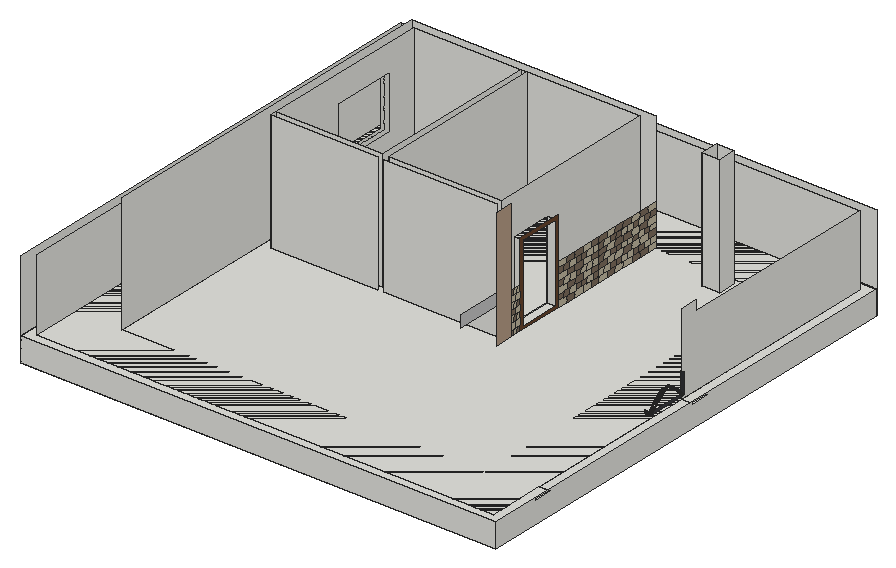
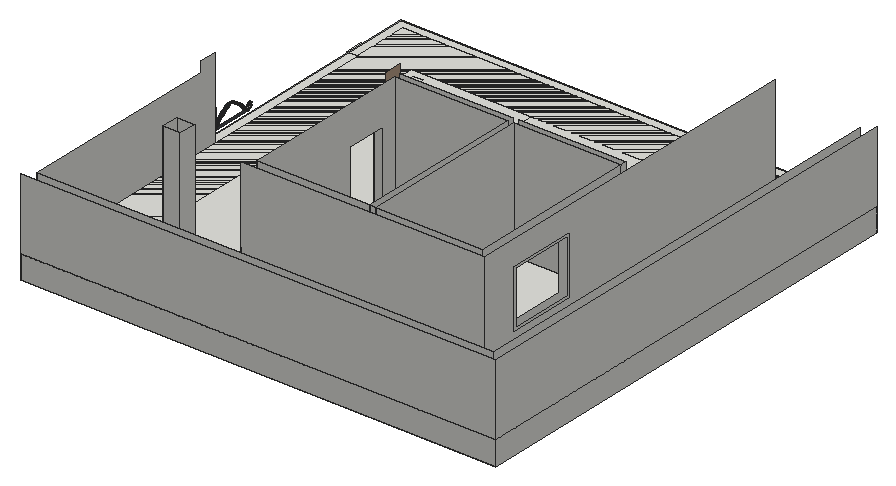
# SketchUp Ruby script. Lengths in inches.
U = 1.inch
M = Sketchup.active_model
def pt(a) = Geom::Point3d.new(a.map { |v| v * U })
def face(e, loops, mat)
  f = e.add_face(loops[0].map { |a| pt(a) })
  loops[1..].each { |l| e.add_face(l.map { |a| pt(a) }).erase! }
  f.material = f.back_material = mat if mat
  f
end
# faces: each face lists its corners as indices into pts; further lists are holes
def faces(e, pts, list, mat = nil) = list.each { |f| face(e, (f[0].is_a?(Array) ? f : [f]).map { |l| l.map { |i| pts[i] } }, mat) }
# xy, xz, yz: faces in a plane at the given z, y or x. An outline is a flat list of corners, or four numbers for a rectangle; further outlines are holes
def ring(l) = l.size == 4 ? [[l[0], l[1]], [l[2], l[1]], [l[2], l[3]], [l[0], l[3]]] : l.each_slice(2).to_a
def flat(e, list, mat, &to3) = list.each { |f| face(e, (f[0].is_a?(Array) ? f : [f]).map { |l| ring(l).map { |u, v| to3.(u, v) } }, mat) }
def xy(e, z, list, mat = nil) = flat(e, list, mat) { |x, y| [x, y, z] }
def xz(e, y, list, mat = nil) = flat(e, list, mat) { |x, z| [x, y, z] }
def yz(e, x, list, mat = nil) = flat(e, list, mat) { |y, z| [x, y, z] }
def lines(e, pts, list) = list.each { |a, b| e.add_line(pt(pts[a]), pt(pts[b])) }
# prism: a flat outline (further loops are holes) pulled along v
def prism(e, loops, v, mat = nil)
  f = face(e, loops, mat); d = Geom::Vector3d.new(v.map { |x| x * U })
  f.pushpull(f.normal.samedirection?(d) ? d.length : -d.length)
end
def box(e, o, s, mat = nil) = prism(e, [[o, [o[0] + s[0], o[1], o[2]], [o[0] + s[0], o[1] + s[1], o[2]], [o[0], o[1] + s[1], o[2]]]], [0, 0, s[2]], mat)
def at(x, y, z, deg = 0) = Geom::Transformation.translation(pt([x, y, z])) * Geom::Transformation.rotation(ORIGIN, Z_AXIS, deg.degrees)
def axes(o, x, y, z) = Geom::Transformation.new([*x, 0, *y, 0, *z, 0, *pt(o).to_a, 1])
def part(name) = M.definitions.add(name)
# library, detail: a bought-in or finely detailed component or shape, given as its bounding box
def library(name, o, s) = part(name).tap { |d| box(d.entities, o, s) }
def detail(e, o, s) = box(e.add_group.entities, o, s)
def put(e, d, t, mat = nil) = e.add_instance(d, t).tap { |i| i.material = mat if mat }
def group(e, t, mat = nil) = e.add_group.tap { |g| g.transformation = t; g.material = mat if mat }.entities
root = M.entities
M.materials.add("Brick_05_1K").color = [195, 185, 161]
M.materials.add("Brick_20_1K").color = [181, 156, 133]
M.materials.add("Brick_20_1K1").color = [126, 109, 93]
M.materials.add("M02_Ash_Whisper").color = [196, 196, 196]
M.materials.add("ThomThom - Buttons1").color = [48, 49, 53]
M.materials.add("Wood_Veneer_15_1K").color = [103, 69, 45]
xy(root,0,[[0,0,480,480]])
xy(root,24,[[0,0,0,480,480,480,480,264,482,264,482,246,471,246,471,471,9,471,9,9,471,9,471,66,482,66,482,48,480,48,480,0],[0,0,480,0,480,66,471,66,471,246,480,246,480,480,0,480],[[9,9,471,471],[57,57,423,423]],[[303,57,423,423],[369,399,387,417],[405,63,417,81]],[471,66,480,246],
  [66,240,174,414],[180,240,294,414]])
xy(root,27,[[294,255,303,297]])
xy(root,32,[[474,200.6875,477,239.78]],"ThomThom - Buttons1")
xz(root,0,[[0,0,480,24]])
xz(root,234,[[66,24,174,144],[180,24,294,144]])
xz(root,240,[[66,24,174,144],[180,24,294,144]])
xz(root,241,[[474,32,477,53.02]],"ThomThom - Buttons1")
xz(root,255,[[294,27,303,105]])
xz(root,297,[[294,27,303,105]])
xz(root,399,[[369,24,387,144]])
xz(root,414,[[66,24,174,144],[174,24,180,144],[180,24,294,144]])
xz(root,417,[[369,24,387,144]])
xz(root,423,[[57,24,303,144]])
xz(root,471,[[9,24,471,96]])
xz(root,480,[[0,0,480,24],[0,24,480,96]])
yz(root,0,[[0,0,480,24],[0,24,480,96]])
yz(root,9,[[9,24,471,96]])
yz(root,57,[[[57,24,423,144],[315,60,387,120]],[[315,60,387,120],[318,63,384,117]]])
yz(root,66,[[234,24,240,144],[[240,24,414,144],[318,63,384,117]]])
yz(root,174,[[240,24,414,144]])
yz(root,180,[[240,24,414,144]])
yz(root,294,[[[240,24,414,144],[255,27,297,105]]])
yz(root,303,[[244,24,248,30],[300,24,310.25,30],[320.5,24,330.75,30],[330.75,24,341,30],[351.25,24,361.5,30],
  [371.75,24,382,30],[382,24,392.25,30],[412.75,24,423,30],[240,30,246,36],[246,30,252,36],
  [314.47,30,321.71,36],[336.18,30,343.41,36],[350.65,30,357.88,36],[357.88,30,365.12,36],[379.59,30,386.82,36],
  [386.82,30,394.06,36],[408.53,30,415.76,36],[415.76,30,423,36],[240,36,244,42],[248,36,252,42],
  [300,36,310.25,42],[330.75,36,341,42],[361.5,36,371.75,42],[371.75,36,382,42],[392.25,36,402.5,42],
  [402.5,36,412.75,42],[246,42,252,48],[307.24,42,314.47,48],[314.47,42,321.71,48],[328.94,42,336.18,48],
  [336.18,42,343.41,48],[343.41,42,350.65,48],[357.88,42,365.12,48],[379.59,42,386.82,48],[386.82,42,394.06,48],
  [401.29,42,408.53,48],[415.76,42,423,48],[240,48,244,54],[244,48,248,54],[300,48,310.25,54],
  [330.75,48,341,54],[361.5,48,371.75,54],[392.25,48,402.5,54],[412.75,48,423,54],[240,54,246,60],
  [246,54,252,60],[314.47,54,321.71,60],[336.18,54,343.41,60],[343.41,54,350.65,60],[357.88,54,365.12,60],
  [379.59,54,386.82,60],[386.82,54,394.06,60],[401.29,54,408.53,60],[244,60,248,66],[248,60,252,66],
  [300,60,310.25,66],[330.75,60,341,66],[361.5,60,371.75,66],[392.25,60,402.5,66],[412.75,60,423,66]],"Brick_05_1K")
yz(root,303,[[222,24,240,144]],"Brick_20_1K")
yz(root,303,[[240,24,244,30],[248,24,252,30],[310.25,24,320.5,30],[341,24,351.25,30],[361.5,24,371.75,30],
  [392.25,24,402.5,30],[402.5,24,412.75,30],[300,30,307.24,36],[307.24,30,314.47,36],[321.71,30,328.94,36],
  [328.94,30,336.18,36],[343.41,30,350.65,36],[365.12,30,372.35,36],[372.35,30,379.59,36],[394.06,30,401.29,36],
  [401.29,30,408.53,36],[244,36,248,42],[310.25,36,320.5,42],[320.5,36,330.75,42],[341,36,351.25,42],
  [351.25,36,361.5,42],[382,36,392.25,42],[412.75,36,423,42],[240,42,246,48],[300,42,307.24,48],
  [321.71,42,328.94,48],[350.65,42,357.88,48],[365.12,42,372.35,48],[372.35,42,379.59,48],[394.06,42,401.29,48],
  [408.53,42,415.76,48],[248,48,252,54],[310.25,48,320.5,54],[320.5,48,330.75,54],[341,48,351.25,54],
  [351.25,48,361.5,54],[371.75,48,382,54],[382,48,392.25,54],[402.5,48,412.75,54],[300,54,307.24,60],
  [307.24,54,314.47,60],[321.71,54,328.94,60],[328.94,54,336.18,60],[350.65,54,357.88,60],[365.12,54,372.35,60],
  [372.35,54,379.59,60],[394.06,54,401.29,60],[408.53,54,415.76,60],[415.76,54,423,60],[240,60,244,66],
  [310.25,60,320.5,66],[320.5,60,330.75,66],[341,60,351.25,66],[351.25,60,361.5,66],[371.75,60,382,66],
  [382,60,392.25,66],[402.5,60,412.75,66]],"Brick_20_1K1")
yz(root,303,[[177,60,222,72]],"M02_Ash_Whisper")
yz(root,303,[[[252,24,300,108],[255,27,297,105]]],"Wood_Veneer_15_1K")
yz(root,369,[[399,24,417,144]])
yz(root,387,[[399,24,417,144]])
yz(root,471,[[246,24,246,106,264,106,264,96,471,96,471,24]])
yz(root,480,[[0,0,480,24]])
p = [[477,198.63,32],[477,197.29,33.67],[474,197.29,33.67],[474,198.63,32],[477,201.49,33],[477,200.6875,32],
  [474,200.6875,32],[474,201.49,33],[477,239.78,32],[477,239.07,33],[474,239.07,33],[474,239.78,32],
  [477,239.87,33.6],[477,241,32],[474,241,32],[474,239.87,33.6],[477,199.27,32.78],[477,199.66,32.25],
  [474,199.66,32.25],[474,199.27,32.78],[477,200.05,32.78],[474,200.05,32.78],[477,198.67,33.55],[474,198.67,33.55],
  [477,200.65,33.55],[474,200.65,33.55],[477,202.03,33.67],[474,202.03,33.67],[477,237.9,34.52],[474,237.9,34.52],
  [477,198.0625,34.3],[474,198.0625,34.3],[477,201.26,34.3],[474,201.26,34.3],[477,238.68,35.15],[474,238.68,35.15],
  [477,196.68,34.4],[474,196.68,34.4],[477,202.64,34.4],[474,202.64,34.4],[477,197.4375,35.05],[474,197.4375,35.05],
  [477,201.88,35.05],[474,201.88,35.05],[477,196.05,35.12],[474,196.05,35.12],[477,203.27,35.12],[474,203.27,35.12],
  [477,236.67,36],[474,236.67,36],[477,196.8,35.78],[474,196.8,35.78],[477,202.52,35.78],[474,202.52,35.78],
  [477,195.41,35.83],[474,195.41,35.83],[477,203.91,35.83],[474,203.91,35.83],[477,237.43,36.65],[474,237.43,36.65],
  [477,196.15,36.51],[474,196.15,36.51],[477,203.17,36.51],[474,203.17,36.51],[477,204.56,36.53],[474,204.56,36.53],
  [477,235.39,37.42],[474,235.39,37.42],[477,195.49,37.22],[474,195.49,37.22],[477,203.83,37.22],[474,203.83,37.22],
  [477,205.22,37.22],[474,205.22,37.22],[477,236.125,38.11],[474,236.125,38.11],[477,194.81,37.92],[474,194.81,37.92],
  [477,204.51,37.92],[474,204.51,37.92],[477,205.9,37.89],[474,205.9,37.89],[477,234.06,38.8],[474,234.06,38.8],
  [477,205.2,38.6],[474,205.2,38.6],[477,206.59,38.55],[474,206.59,38.55],[477,234.76,39.51],[474,234.76,39.51],
  [477,205.9,39.28],[474,205.9,39.28],[477,207.29,39.2],[474,207.29,39.2],[477,232.67,40.12],[474,232.67,40.12],
  [477,208,39.84],[474,208,39.84],[477,206.61,39.94],[474,206.61,39.94],[477,233.34,40.85],[474,233.34,40.85],
  [477,208.72,40.46],[474,208.72,40.46],[477,207.34,40.59],[474,207.34,40.59],[477,231.23,41.38],[474,231.23,41.38],
  [477,209.45,41.07],[474,209.45,41.07],[477,208.07,41.22],[474,208.07,41.22],[477,231.875,42.15],[474,231.875,42.15],
  [477,210.2,41.67],[474,210.2,41.67],[477,208.82,41.85],[474,208.82,41.85],[477,229.74,42.59],[474,229.74,42.59],
  [477,210.95,42.25],[474,210.95,42.25],[477,209.58,42.46],[474,209.58,42.46],[477,230.36,43.38],[474,230.36,43.38],
  [477,211.72,42.82],[474,211.72,42.82],[477,210.35,43.05],[474,210.35,43.05],[477,228.21,43.74],[474,228.21,43.74],
  [477,212.49,43.38],[474,212.49,43.38],[477,211.13,43.63],[474,211.13,43.63],[477,213.28,43.92],[474,213.28,43.92],
  [477,228.79,44.55],[474,228.79,44.55],[477,211.92,44.2],[474,211.92,44.2],[477,226.63,44.83],[474,226.63,44.83],
  [477,214.07,44.45],[474,214.07,44.45],[477,212.72,44.75],[474,212.72,44.75],[477,214.88,44.96],[474,214.88,44.96],
  [477,227.1875,45.66],[474,227.1875,45.66],[477,213.53,45.29],[474,213.53,45.29],[477,225.02,45.86],[474,225.02,45.86],
  [477,215.69,45.46],[474,215.69,45.46],[477,214.35,45.8125],[474,214.35,45.8125],[477,216.51,45.95],[474,216.51,45.95],
  [477,225.54,46.71],[474,225.54,46.71],[477,215.18,46.32],[474,215.18,46.32],[477,217.34,46.42],[474,217.34,46.42],
  [477,223.36,46.82],[474,223.36,46.82],[477,216.01,46.8125],[474,216.01,46.8125],[477,218.18,46.87],[474,218.18,46.87],
  [477,223.84,47.69],[474,223.84,47.69],[477,216.86,47.29],[474,216.86,47.29],[477,221.67,47.72],[474,221.67,47.72],
  [477,219.03,47.31],[474,219.03,47.31]]
faces(root,p,[[0,1,2,3],[4,5,6,7],[8,9,10,11],[16,17,18,19],[17,20,21,18],[22,16,19,23],[20,24,25,21],[26,4,7,27],
  [9,28,29,10],[30,22,23,31],[24,32,33,25],[1,36,37,2],[38,26,27,39],[40,30,31,41],[32,42,43,33],[36,44,45,37],
  [46,38,39,47],[28,48,49,29],[50,40,41,51],[42,52,53,43],[44,54,55,45],[56,46,47,57],[60,50,51,61],[52,62,63,53],
  [64,56,57,65],[48,66,67,49],[68,60,61,69],[62,70,71,63],[72,64,65,73],[76,68,69,77],[70,78,79,71],[80,72,73,81],
  [66,82,83,67],[78,84,85,79],[86,80,81,87],[84,90,91,85],[92,86,87,93],[82,94,95,83],[96,92,93,97],[90,98,99,91],
  [102,96,97,103],[98,104,105,99],[94,106,107,95],[108,102,103,109],[104,110,111,105],[114,108,109,115],[110,116,117,111],[106,118,119,107],
  [120,114,115,121],[116,122,123,117],[126,120,121,127],[122,128,129,123],[118,130,131,119],[132,126,127,133],[128,134,135,129],[136,132,133,137],
  [134,140,141,135],[130,142,143,131],[144,136,137,145],[140,146,147,141],[148,144,145,149],[146,152,153,147],[142,154,155,143],[156,148,149,157],
  [152,158,159,153],[160,156,157,161],[158,164,165,159],[166,160,161,167],[154,168,169,155],[164,170,171,165],[172,166,167,173],[170,176,177,171],
  [168,178,179,169],[180,172,173,181]])
faces(root,p,[[12,13,14,15],[34,12,15,35],[58,34,35,59],[74,58,59,75],[88,74,75,89],[100,88,89,101],[112,100,101,113],[124,112,113,125],
  [138,124,125,139],[150,138,139,151],[162,150,151,163],[174,162,163,175]],"ThomThom - Buttons1")
